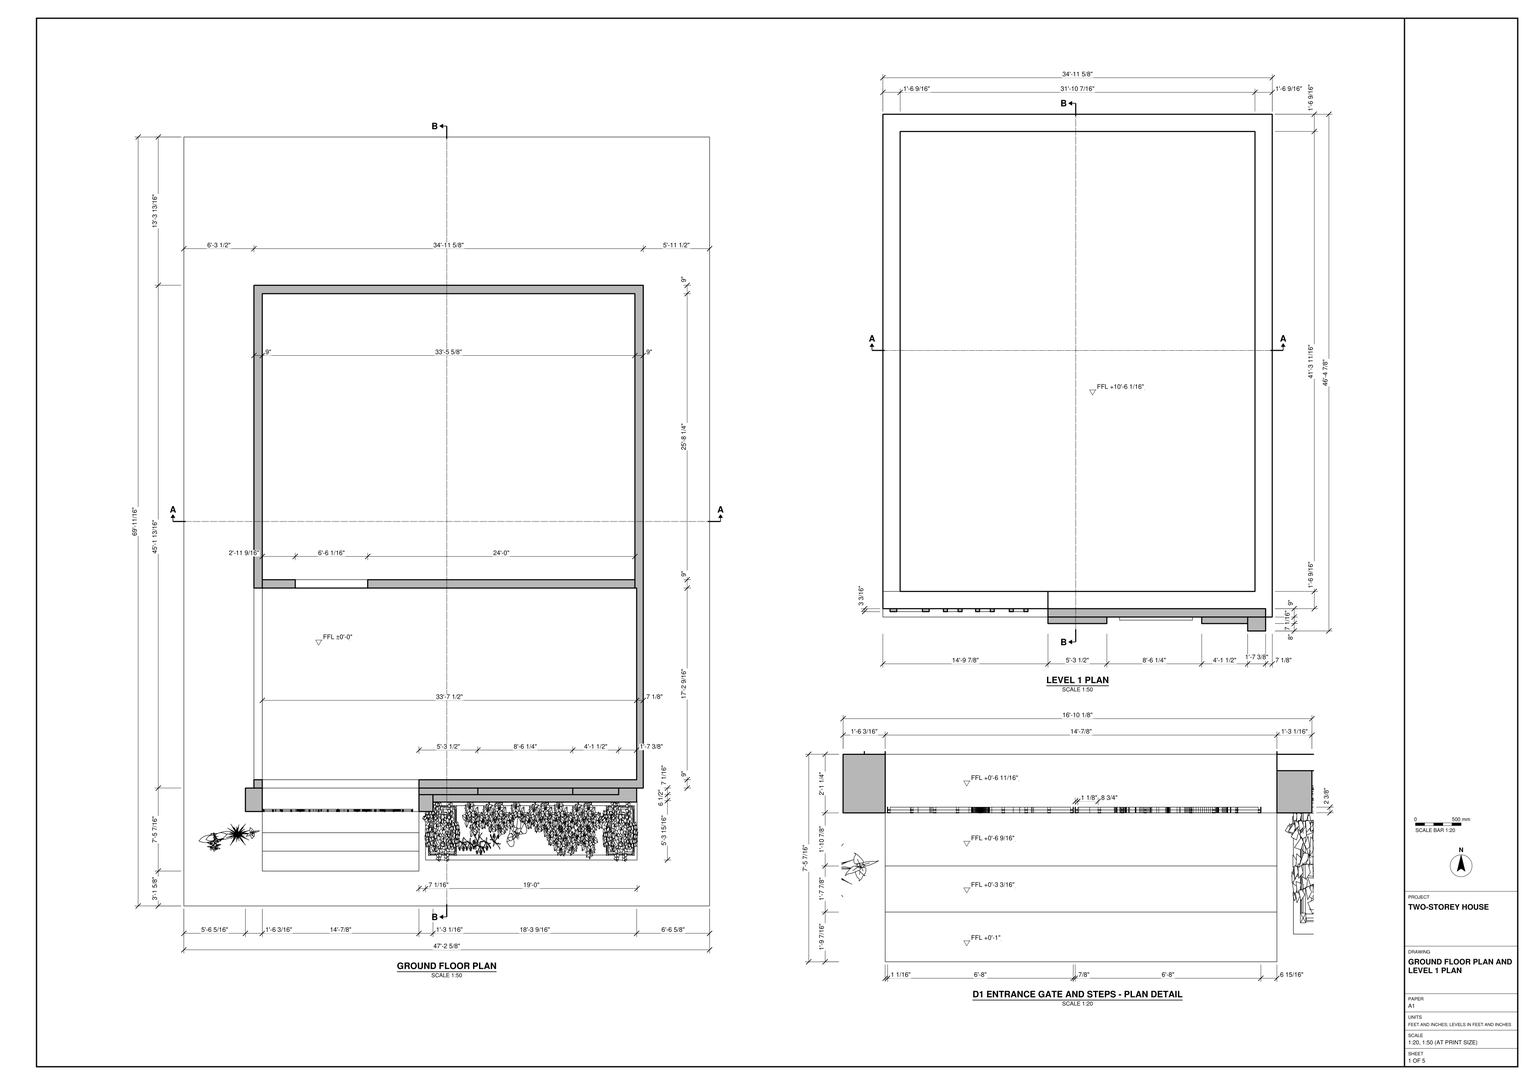
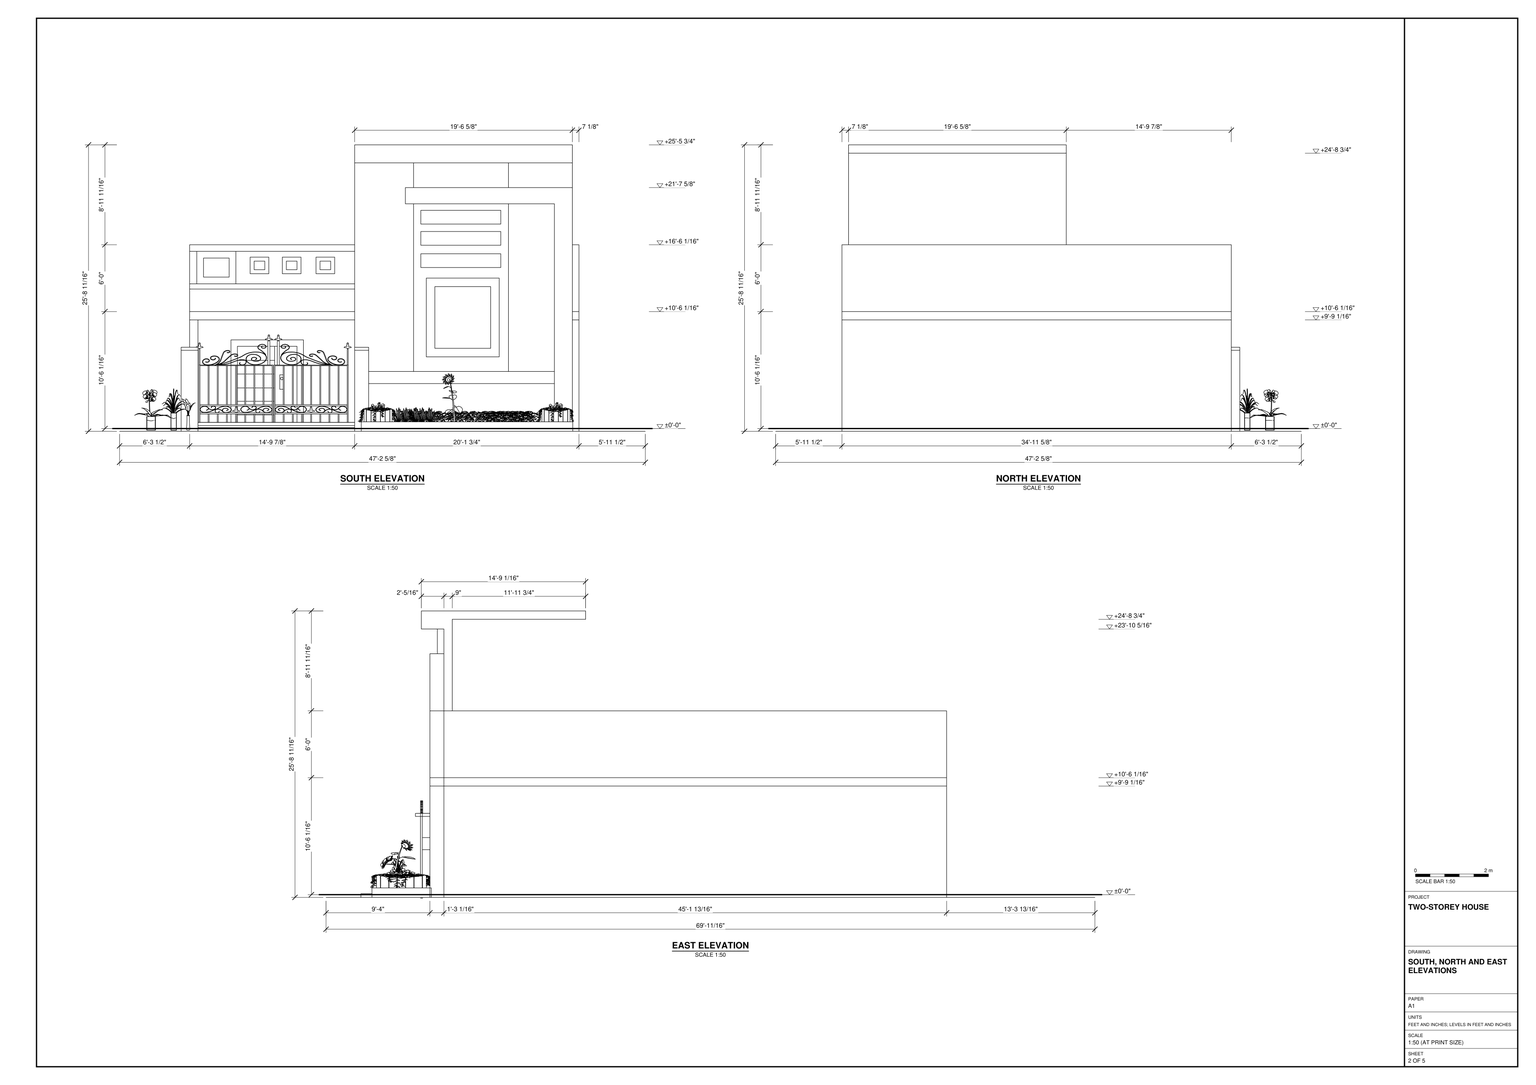
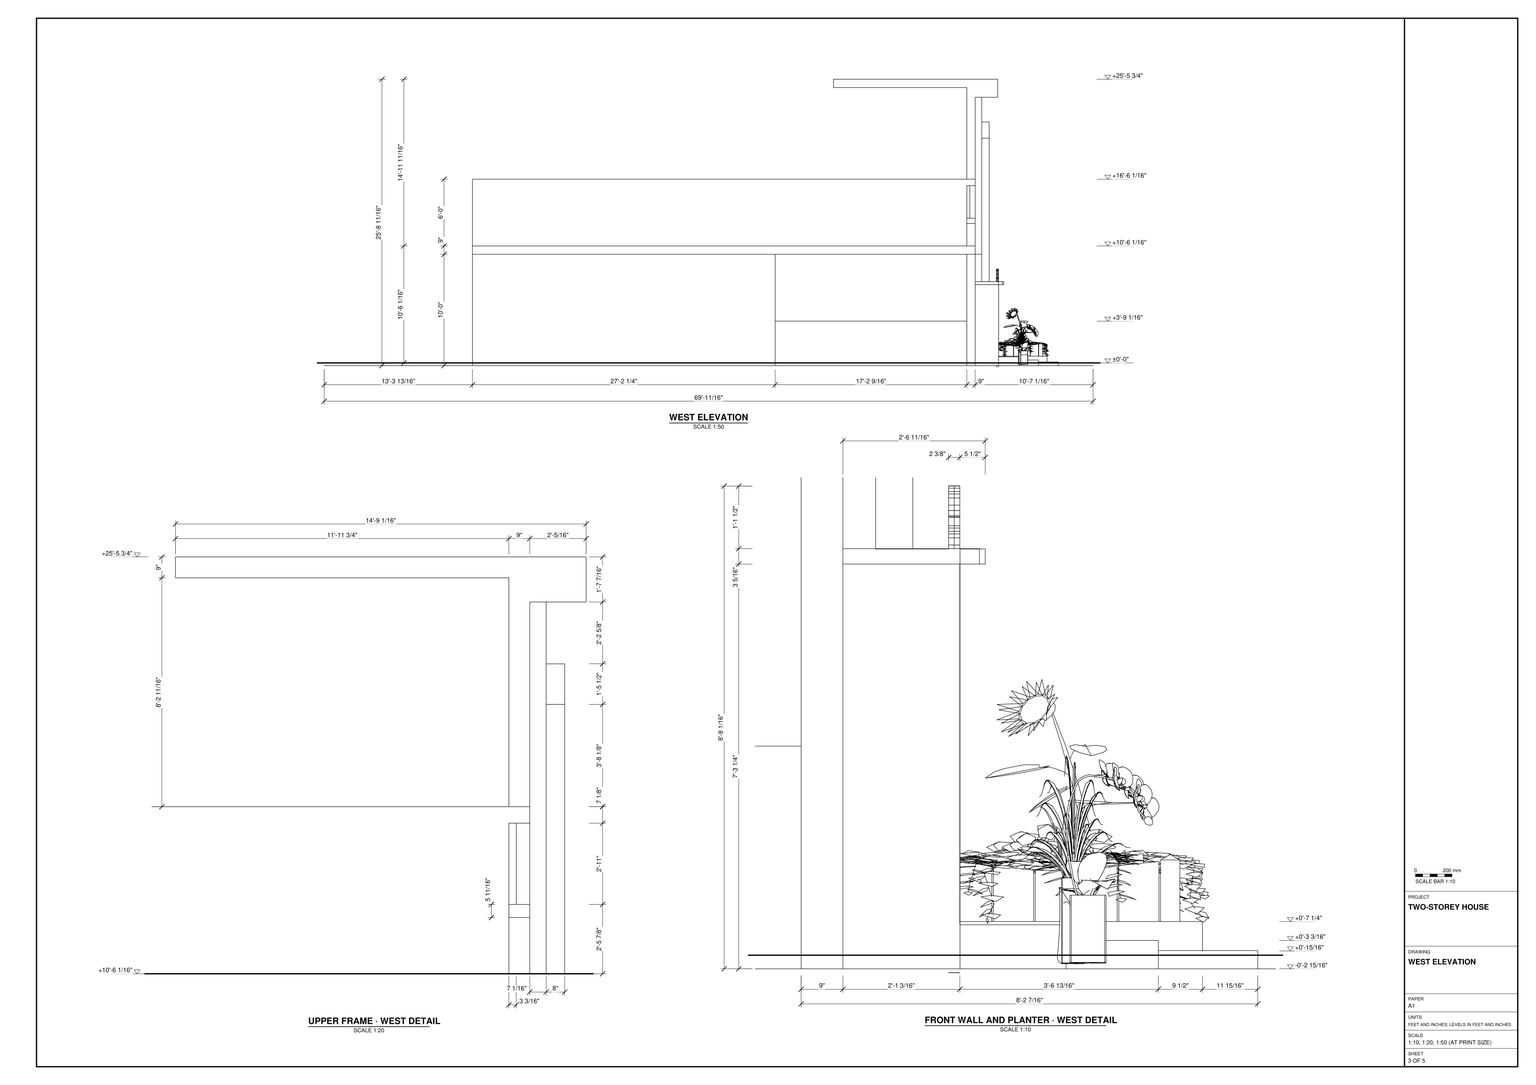
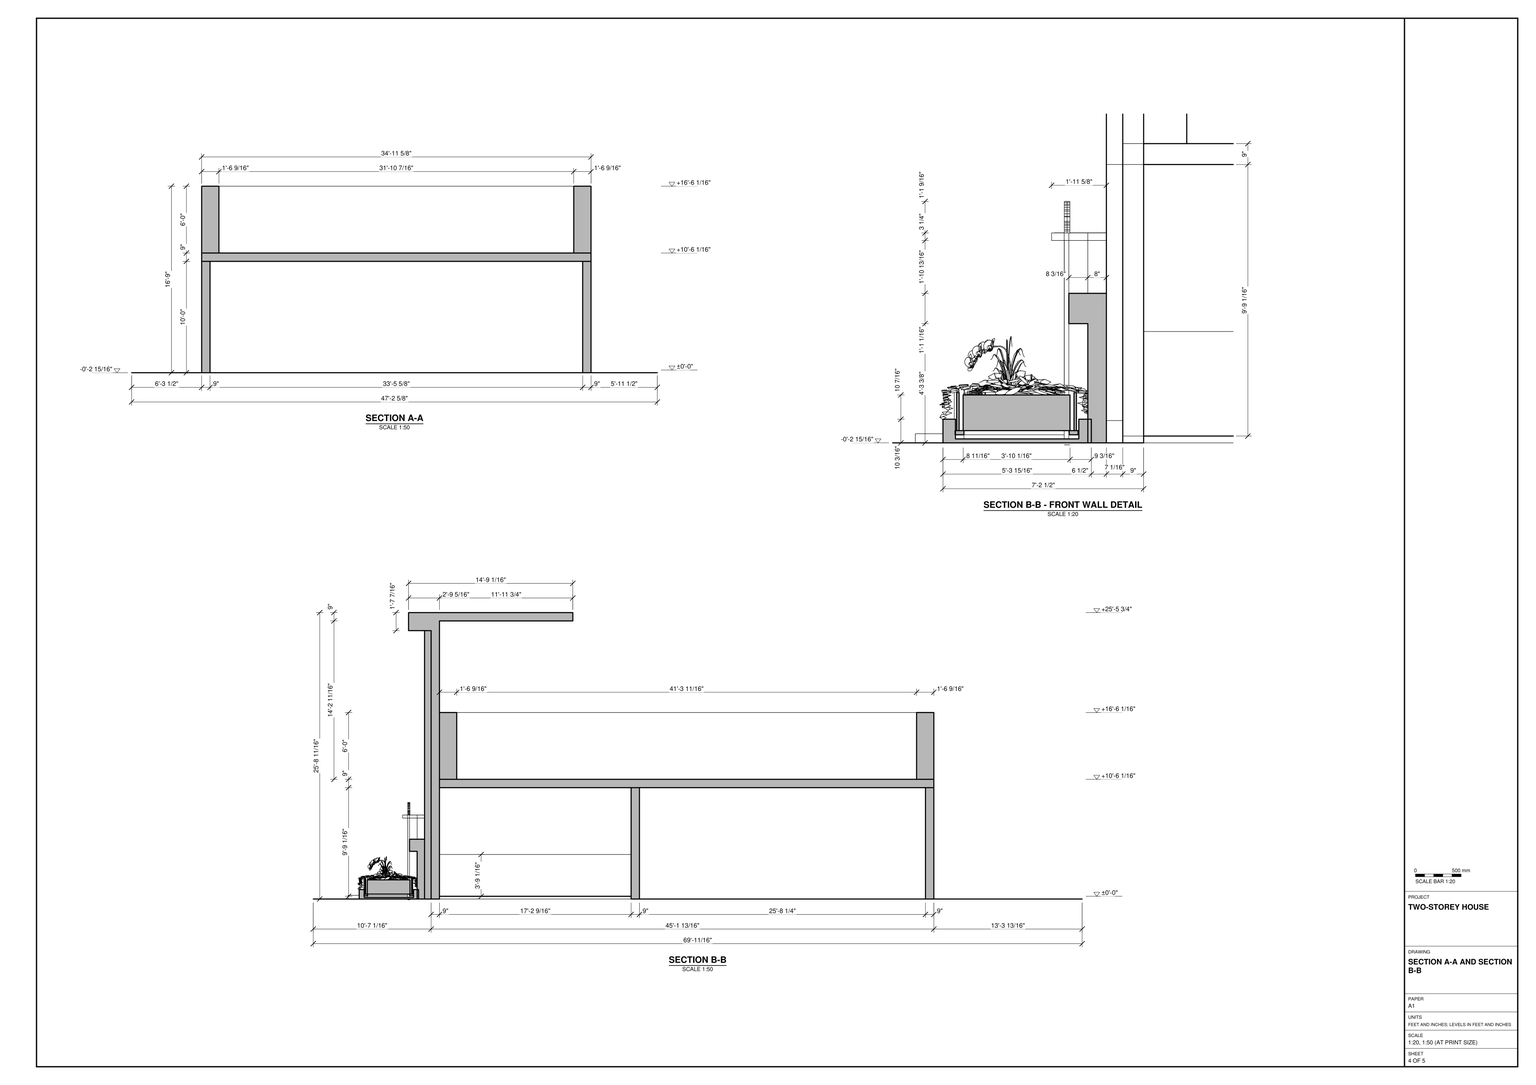
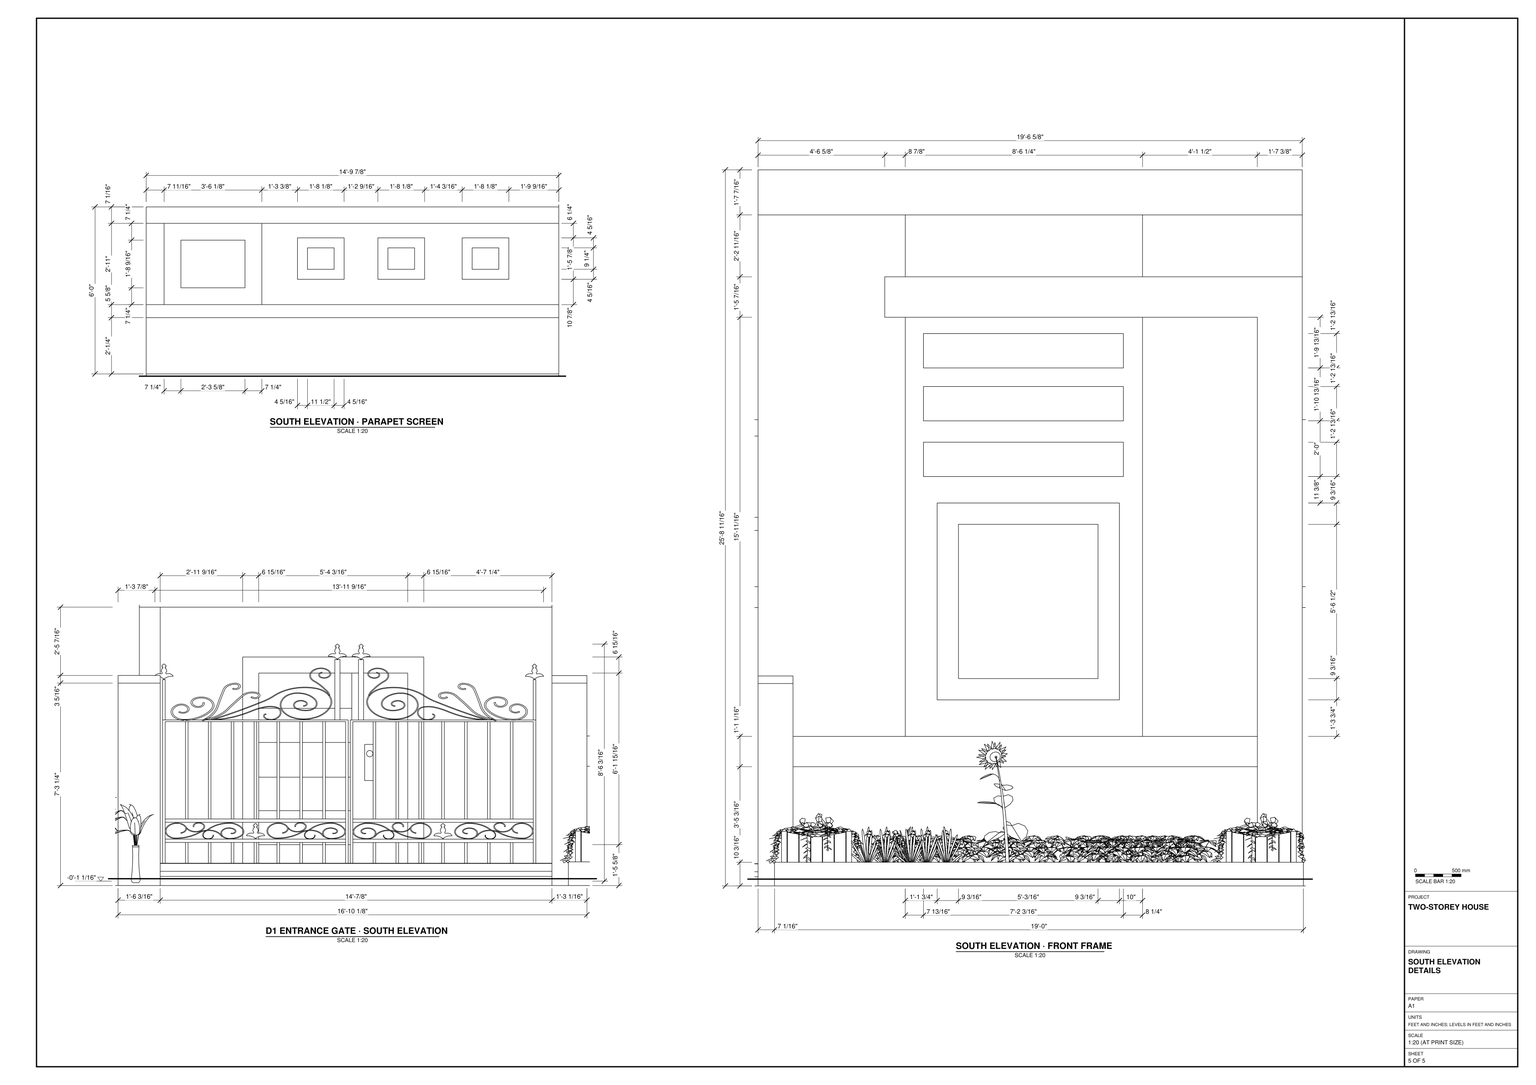
Build the house and its rectangular site in SketchUp from task_files/diagram_01.pdf. Work in feet and inches. The overall model is 47'-2 5/8" wide, 69'-11/16" deep and 25'-8 11/16" high. Set the ground floor at ±0'-0" and the upper floor at +10'-6 1/16".

Use the ground-floor plan to locate the house within the site. Model the rear enclosure, the cross wall with its offset doorway, and the entrance area in front of it. Follow the wall thicknesses as drawn, including the 9" walls around the rear enclosure. Form the upper slab and its raised perimeter, keeping the long side and rear elevations plain as shown.

Use the south elevation to set out the two different sides of the frontage. On the left, build the broad entrance steps, gateposts and paired gate leaves beneath the low band of framed panels. On the right, model the taller frame with its projecting flat roof, layered uprights, large framed panel and horizontal panels above. Use the west details to set the roof projection and the offsets between the front wall, planter and steps. Decor and loose items, including the planting, may be any suitable library components.

Keep walls, slabs, roof, gate and each furniture or joinery piece in separate groups or components, and use components for repeated parts. Save one SketchUp model as output_files/two_storey_house_with_a_stepped_entrance_and_front_gate.skp.

# SketchUp Ruby script. Lengths in inches.
U = 1.inch
M = Sketchup.active_model
def pt(a) = Geom::Point3d.new(a.map { |v| v * U })
def face(e, loops, mat)
  f = e.add_face(loops[0].map { |a| pt(a) })
  loops[1..].each { |l| e.add_face(l.map { |a| pt(a) }).erase! }
  f.material = f.back_material = mat if mat
  f
end
# faces: each face lists its corners as indices into pts; further lists are holes
def faces(e, pts, list, mat = nil) = list.each { |f| face(e, (f[0].is_a?(Array) ? f : [f]).map { |l| l.map { |i| pts[i] } }, mat) }
# xy, xz, yz: faces in a plane at the given z, y or x. An outline is a flat list of corners, or four numbers for a rectangle; further outlines are holes
def ring(l) = l.size == 4 ? [[l[0], l[1]], [l[2], l[1]], [l[2], l[3]], [l[0], l[3]]] : l.each_slice(2).to_a
def flat(e, list, mat, &to3) = list.each { |f| face(e, (f[0].is_a?(Array) ? f : [f]).map { |l| ring(l).map { |u, v| to3.(u, v) } }, mat) }
def xy(e, z, list, mat = nil) = flat(e, list, mat) { |x, y| [x, y, z] }
def xz(e, y, list, mat = nil) = flat(e, list, mat) { |x, z| [x, y, z] }
def yz(e, x, list, mat = nil) = flat(e, list, mat) { |y, z| [x, y, z] }
def lines(e, pts, list) = list.each { |a, b| e.add_line(pt(pts[a]), pt(pts[b])) }
# prism: a flat outline (further loops are holes) pulled along v
def prism(e, loops, v, mat = nil)
  f = face(e, loops, mat); d = Geom::Vector3d.new(v.map { |x| x * U })
  f.pushpull(f.normal.samedirection?(d) ? d.length : -d.length)
end
def box(e, o, s, mat = nil) = prism(e, [[o, [o[0] + s[0], o[1], o[2]], [o[0] + s[0], o[1] + s[1], o[2]], [o[0], o[1] + s[1], o[2]]]], [0, 0, s[2]], mat)
def at(x, y, z, deg = 0) = Geom::Transformation.translation(pt([x, y, z])) * Geom::Transformation.rotation(ORIGIN, Z_AXIS, deg.degrees)
def axes(o, x, y, z) = Geom::Transformation.new([*x, 0, *y, 0, *z, 0, *pt(o).to_a, 1])
def part(name) = M.definitions.add(name)
# library, detail: a bought-in or finely detailed component or shape, given as its bounding box
def library(name, o, s) = part(name).tap { |d| box(d.entities, o, s) }
def detail(e, o, s) = box(e.add_group.entities, o, s)
def put(e, d, t, mat = nil) = e.add_instance(d, t).tap { |i| i.material = mat if mat }
def group(e, t, mat = nil) = e.add_group.tap { |g| g.transformation = t; g.material = mat if mat }.entities
root = M.entities
M.materials.add("[Blinds Wood Natural]").color = [167, 145, 74]
M.materials.add("[Color C01]").color = [255, 229, 204]
M.materials.add("[Color C03]").color = [255, 178, 101]
M.materials.add("[Color C04]").color = [255, 153, 50]
M.materials.add("[Color D03]").color = [255, 216, 101]
M.materials.add("[Color D04]").color = [255, 204, 50]
M.materials.add("[Formica Graystone]").color = [149, 146, 135]
M.materials.add("[Formica Laminate Dark]").color = [50, 53, 60]
M.materials.add("[Formica Speckled Grey]").color = [94, 105, 111]
M.materials.add("[Translucent Glass Sky Reflection]").color = [126, 138, 183]
M.materials["[Translucent Glass Sky Reflection]"].alpha = 0.52
M.materials.add("[Wood Bamboo]").color = [177, 105, 43]
M.materials.add("[Wood Board Cork]").color = [215, 201, 115]
M.materials.add("[Wood Veneer 01]").color = [120, 70, 37]
M.materials.add("bottom").color = [37, 104, 50]
c1 = library("gate",[-17.08,19.83,-10.33],[162.44,1,145.04])
c2 = library("Planter_Wood_Square",[-12.51,-6.53,0],[58.51,52.32,45.58])
c3 = library("Plant_Sunflower",[-13.8,-15.43,0],[27.09,16.85,64.87])
c4 = part("Lg Broken Leaf")
p = [[0.72,6.4,1.375],[1.32,6.4,1.375],[1.31,6.44,1.32],[1.02,7.29,0],[0.73,6.44,1.32],[0.5,5.3,2.66],
  [1.54,5.3,2.66],[1.53,5.35,2.61],[1.4375,5.9,1.96],[0.6,5.9,1.96],[0.51,5.35,2.61],[0.44,4.6875,3.23],
  [0.41,4.02,3.84],[1.63,4.02,3.84],[1.6,4.6875,3.23],[0.43,2.57,4.9],[1.61,2.57,4.9],[1.63,3.22,4.43],
  [0.41,3.22,4.43],[0.65,0.97,5.83],[1.39,0.97,5.83],[1.47,1.4,5.58],[1.54,1.9,5.29],[1.6,2.41,5],
  [0.44,2.41,5],[0.5,1.9,5.29],[0.57,1.4,5.58],[1.02,0.33,6.11]]
faces(c4.entities,p,[[0,1,2,3,4],[5,6,7,8,1,0,9,10],[6,5,11,12,13,14],[15,16,17,13,12,18],[19,20,21,22,23,16,15,24,25,26],[19,27,20]],"bottom")
c5 = part("stalk")
xy(c5.entities,13.2,[[0.11,0.17,0.11,0.29,0,0.23]])
p = [[0.8,0,0],[0.3,0,7.2],[0.05,0.15,7.2],[0.64,0.09,0],[0.8,0.18,0],[0.3,0.29,7.2],
  [0.11,0.17,13.2],[0,0.23,13.2],[0.11,0.29,13.2]]
faces(c5.entities,p,[[0,1,2,3],[0,4,5,1],[3,2,5,4],[1,6,7,2],[1,5,8,6],[2,7,8,5]])
c6 = part("petal\#1")
p = [[0.62,0.42,-0.27],[0.71,0.28,-0.07],[0.72,0.84,-0.07],[0.62,0.7,-0.27],[1,0,0.21],[1,1.12,0.2],
  [1.53,1.12,0.4375],[1.53,0,0.4375],[1.53,0.56,0.4375],[1.99,0.28,0.3],[2.23,0.42,0.23],[2.23,0.7,0.22],
  [1.99,0.84,0.3],[1.76,0.79,0.37],[1.76,0.33,0.37]]
faces(c6.entities,p,[[0,1,2,3],[1,4,5,2],[6,5,4,7,8],[9,10,11,12,13,8,14],[14,8,7,9],[6,8,13,12]])
c7 = part("petal\#2")
p = [[1.12,0.18,-0.52],[1.09,-0.07,-0.2],[1.09,0.58,-0.2],[1.12,0.37,-0.52],[1.25,-0.26,0.16],[1.25,0.78,0.16],
  [1.64,0.81,0.44],[1.64,-0.23,0.44],[1.64,0.36,0.44],[1.875,0.2,0.36],[2.24,0,0.23],[2.34,0.26,0.2],
  [2.34,0.45,0.2],[2.08,0.61,0.29],[1.875,0.51,0.36]]
faces(c7.entities,p,[[0,1,2,3],[1,4,5,2],[6,5,4,7,8],[9,8,7,10],[10,11,12,13,14,8,9],[6,8,14,13]])
c8 = part("flower\#1")
put(c8.entities,c6,axes([2.11,0.17,0.22],[-0.04332,0.67288,0.31447],[-0.79297,-0.00158,-0.10584],[-0.09505,-0.34133,0.71726]))
put(c8.entities,c6,axes([1.96,3.15,0.77],[-0.34058,-0.53026,-0.04745],[0.67203,-0.43351,0.02099],[-0.07223,-0.05636,1.14835]))
put(c8.entities,c7,axes([1.875,2.15,2.86],[-0.19209,-0.10227,-0.76975],[0.18918,-0.78348,0.05688],[0.7612,0.16839,-0.21233]))
put(c8.entities,c7,axes([-0.27,1.75,2.2],[0.7458,-0.1672,-0.4029],[0.09529,0.84119,-0.17269],[-0.42568,-0.10463,-0.74454]))
put(c8.entities,c7,axes([1.35,1,3.03],[0.21021,0.29303,-0.80271],[-0.84848,0.16975,-0.16023],[-0.10149,-0.81223,-0.32308]))
put(c8.entities,c6,axes([-0.01,1.74,0.14],[0.65005,-0.20903,0.29542],[0.19101,0.76714,0.12251],[-0.33903,-0.0312,0.72394]))
c9 = part("flower all")
put(c9.entities,c5,axes([1.5,1.42,0],[1,0,0],[0,1,0],[0,0,0.95]))
put(c9.entities,c8,axes([-0.1875,-0.26,11.36],[1.15,0,0],[0,1.15,0],[0,0,1.15]))
c10 = part("Plant_Iris")
put(c10.entities,c4,axes([2.34,6.11,0.91],[-0.7307,0.19579,0],[-0.22806,-0.85114,-0.14272],[-0.13461,-0.50236,3.2111]))
put(c10.entities,c4,axes([-1.55,-5.13,1.15],[0.73882,-0.13929,-0.08363],[0.1194,0.7313,-0.16322],[0.43446,0.57278,2.88421]),"bottom")
put(c10.entities,c4,axes([2.25,3.63,0.45],[-0.67969,0.25481,0.21297],[-0.22484,-0.52301,-0.09181],[0.54964,-0.68886,2.5783]),"bottom")
put(c10.entities,c4,axes([0.97,5.42,1.15],[-0.75102,0.03511,-0.08363],[-0.01646,-0.7408,-0.16322],[-0.36512,-0.65382,3.00438]),"bottom")
put(c10.entities,c4,axes([-1.78,-3.31,-0.01],[0.47543,-0.10678,0.47549],[0.18828,0.47676,-0.08118],[-0.92661,0.54451,1.04877]),"bottom")
put(c10.entities,c9,axes([2.89,-2.41,-0.46],[-0.34687,1.29454,0.20029],[-1.30891,-0.35072,0],[0.05184,-0.19347,1.3402]))
put(c10.entities,c4,axes([-1.58,-3.78,0.45],[0.70854,-0.15773,0.21297],[0.14986,0.54921,-0.09181],[-0.64016,0.60566,2.5783]),"bottom")
put(c10.entities,c4,axes([1.58,3.45,1.03],[-0.55594,0.20323,-0.33638],[-0.13288,-0.49532,-0.07964],[-1.26871,0.00294,2.09858]),"bottom")
put(c10.entities,c4,axes([-1.84,-3.14,0.82],[0.51728,-0.26469,-0.35481],[0.18828,0.47676,-0.08118],[0.9646,-0.12552,1.4999]),"bottom")
put(c10.entities,c4,axes([-1.95,-3.09,0.74],[0.55657,-0.28236,-0.27208],[0.20053,0.47201,-0.07964],[1.04737,-0.07102,2.21622]),"bottom")
put(c10.entities,c9,axes([2.04,-1.8125,0.13],[-0.26709,0.99679,0.15423],[-0.97505,-0.21431,-0.30344],[-0.2582,-0.22179,0.98634]))
c11 = part("leaf\#2")
p = [[2.22,5.43,0.5],[2.22,4.99,0.65],[2.22,3.75,0.8],[2.22,1.875,0.75],[2.22,0,0.5]]
lines(c11.entities,p,[[0,1],[1,2],[2,3],[3,4]])
g1 = group(c11.entities,at(-0.85,1.38,-0.53))
p = [[1.95,0.49,1.28],[3.0625,-1.38,1.03],[4.17,0.49,1.28],[4.89,3.61,1.18],[3.0625,4.05,1.03],[1.23,3.61,1.18],
  [5.28,2.37,1.33],[0.85,2.37,1.33],[4.09,0.37,1.26],[3.0625,5.5,0.53]]
faces(g1,p,[[0,1,2],[3,4,5],[6,7,5,3],[6,2,0,7]])
lines(g1,p,[[2,8],[4,9]])
c12 = part("stem")
p = [[0.07,0.07,0],[0.18,-0.6,6.17],[0.15,-0.52,6.17],[0,0.23,0],[0.22,0,0],[0.26,-0.63,6.17],
  [0.38,0.07,0],[0.34,-0.6,6.17],[0.45,0.23,0],[0.375,-0.52,6.17],[0.18,-0.44,6.17],[0.07,0.38,0],
  [0.38,0.38,0],[0.34,-0.44,6.17],[0.22,0.45,0],[0.26,-0.41,6.17],[0.3,0.36,14.04],[0.3,0.37,14.04],
  [0.31,0.36,14.04],[0.32,0.37,14.04],[0.3125,0.36,14.04],[0.3,0.375,14.04],[0.3125,0.375,14.04],[0.31,0.375,14.04]]
faces(c12.entities,p,[[0,1,2,3],[0,4,5,1],[6,7,5,4],[6,8,9,7],[3,2,10,11],[8,12,13,9],[14,11,10,15],[14,15,13,12],
  [1,16,17,2],[1,5,18,16],[7,9,19,20],[7,20,18,5],[2,17,21,10],[9,13,22,19],[15,10,21,23],[15,23,22,13]])
c13 = part("Plant_Copperleaf")
put(c13.entities,c11,axes([-5.58,4.88,9.66],[0.029,-0.6438,-0.08473],[0.46185,-0.03917,0.4557],[-0.45646,-0.08053,0.4557]))
put(c13.entities,c11,axes([-5.08,1.59,6.46],[0.32516,-0.5592,0.06373],[0.34931,0.25823,0.48353],[-0.4413,-0.20764,0.4297]))
put(c13.entities,c11,axes([1.03,7.88,12.84],[-0.74201,0.41464,0],[-0.35359,-0.63275,0.44396],[0.21657,0.38756,0.72484]))
put(c13.entities,c11,axes([8.15,-2.85,6.5],[0.20357,0.97906,0],[-0.82181,0.17088,0.54354],[0.53216,-0.11065,0.83938]))
put(c13.entities,c11,axes([-2.45,-8.68,11.21],[0.44862,0.69737,0.18686],[-0.68348,0.33936,0.37442],[0.23259,-0.34787,0.73986]))
put(c13.entities,c11,axes([5.75,-5.02,11.05],[0.73612,0.3986,0.14745],[-0.425,0.6904,0.25539],[0,-0.2949,0.79721]))
put(c13.entities,c11,axes([-9.53,-8.18,10.32],[0.69881,-0.44455,0.19116],[0.26519,0.63267,0.5019],[-0.40477,-0.35298,0.65883]))
put(c13.entities,c11,axes([-3.54,0.82,12.95],[0.59529,0.24687,-0.08473],[-0.12073,0.44751,0.4557],[0.23141,-0.40161,0.4557]))
put(c13.entities,c11,axes([-7.83,6.75,12.84],[-0.07243,-0.84691,0],[0.72233,-0.06177,0.44377],[-0.44215,0.03781,0.72496]))
put(c13.entities,c11,axes([5.33,5.4,7.18],[-0.82339,0.16353,0.1334],[-0.08131,-0.74163,0.40728],[0.19475,0.38176,0.73405]))
put(c13.entities,c11,axes([1.24,4.74,6.1875],[-0.56984,-0.3127,0],[0.2731,-0.49769,0.31658],[-0.1523,0.27754,0.56769]))
put(c13.entities,c11,axes([-7.98,-0.98,12.17],[-0.32199,-0.5173,-0.22633],[0.3682,-0.38989,0.3673],[-0.42807,0.05375,0.48617]))
put(c13.entities,c11,axes([-6.29,1.25,4.06],[0.17169,-0.81932,0.14745],[0.70535,0.22313,0.41856],[-0.44215,0.03781,0.72496]))
put(c13.entities,c11,axes([1.45,5.96,12.73],[-0.5734,-0.62614,-0.04073],[0.6224,-0.57457,0.07055],[-0.07951,0.01777,0.84609]))
put(c13.entities,c11,axes([2.15,3.51,2.68],[-0.74201,0.41464,0],[-0.26708,-0.47794,0.65018],[0.31717,0.56758,0.54751]))
put(c13.entities,c11,axes([-1.77,-7.74,6.875],[0.58011,0.60352,0.14745],[-0.5818,0.45697,0.41856],[0.21792,-0.38658,0.72496]))
put(c13.entities,c11,axes([4.56,3.08,6.68],[-0.50822,0.85524,-0.10132],[-0.77037,-0.39886,0.49743],[0.38501,0.33086,0.86157]))
put(c13.entities,c11,axes([-1.36,-1.16,13.02],[-0.63498,0.48874,0.28361],[-0.49336,-0.68751,0.08018],[0.27549,-0.10472,0.79727]))
put(c13.entities,c12,axes([-0.77,0.55,5.03],[0.06901,0.68185,-0.0317],[-0.56289,0.07487,0.38502],[0.38611,-0.01272,0.56696]))
put(c13.entities,c11,axes([-1.01,-0.89,8.07],[-0.53939,0.35267,-0.08473],[-0.34351,-0.44796,0.32223],[0.11644,0.31217,0.55811]))
put(c13.entities,c11,axes([6.98,3.76,4.09],[-0.72792,0.66854,0.15229],[-0.49329,-0.66488,0.56089],[0.47623,0.33316,0.81376]))
put(c13.entities,c11,axes([-1.09,-1.24,11.25],[0.51443,-0.67666,0],[0.64058,0.487,0.27383],[-0.21799,-0.16573,0.80468]))
put(c13.entities,c11,axes([8.08,1.18,10.18],[-0.40665,0.49996,-0.08473],[-0.39437,-0.24354,0.4557],[0.31876,0.3365,0.4557]))
put(c13.entities,c11,axes([-9.63,-1.83,7.02],[0.07558,-0.84663,0],[0.72197,0.06445,0.44396],[-0.4422,-0.03947,0.72484]))
put(c13.entities,c11,axes([2.71,-1.18,1.48],[0.27025,0.73847,0.14708],[-0.41941,0.01785,0.68101],[0.62535,-0.30716,0.39318]))
put(c13.entities,c12,axes([-0.27,-0.29,-0.05],[1.17914,0.05766,0.21521],[0,1.15911,-0.31058],[-0.2228,0.30518,1.13896]))
put(c13.entities,c11,axes([1.52,0.375,4.23],[-0.45629,0.46292,0.00108],[-0.43266,-0.427,0.23018],[0.16464,0.16086,0.60788]))
put(c13.entities,c11,axes([-7.16,-2.94,2.12],[0.60544,-0.58565,-0.11382],[0.48786,0.39265,0.57473],[-0.34341,-0.4747,0.61582]))
put(c13.entities,c11,axes([-3.79,3.68,3.05],[-0.44676,-0.6045,-0.39686],[0.31657,-0.58291,0.53151],[-0.65015,0.13155,0.53151]))
put(c13.entities,c11,axes([-0.3,8.01,9.4],[-0.82874,0.11809,0.14745],[-0.03086,-0.73916,0.41856],[0.18637,0.40274,0.72496]))
put(c13.entities,c12,axes([-0.79,0.44,2.66],[0.65559,-0.72856,0],[0.60007,0.53997,0.55583],[-0.41317,-0.3718,0.80725]))
put(c13.entities,c11,axes([2.6875,-5.36,4.22],[0.87183,0.48981,0],[-0.39311,0.69971,0.59654],[0.29219,-0.52008,0.80258]))
put(c13.entities,c11,axes([0.09,-5.84,2.26],[0.61933,0.36626,0.45253],[-0.57159,0.50795,0.37117],[-0.11049,-0.57475,0.61641]))
put(c13.entities,c11,axes([-0.51,-1.82,9.55],[0.64288,0.55606,0],[-0.47418,0.54822,0.44396],[0.29044,-0.33578,0.72484]))
put(c13.entities,c11,axes([-3.38,7.24,4.89],[-0.76712,-0.64061,0.03388],[0.46704,-0.52151,0.71407],[-0.43977,0.5636,0.69925]))
c14 = part("Group\#6")
put(c14.entities,c13,at(38.08,13.93,0.15,57.3))
put(c14.entities,c13,at(8.91,14.4,0.15,95.1))
put(c14.entities,c13,at(27.59,12.47,0.15,84.3))
put(c14.entities,c13,at(47.4,9.34,0.15))
put(c14.entities,c13,at(17.4,9.34,0.15))
c15 = part("sledgegarden")
xy(c15.entities,0,[[-83.88,-7.53,144.12,28.47]])
xy(c15.entities,2,[[-80.85,-4.5,-50.62,25.4375],[110.87,-4.5,141.09,25.4375]])
xy(c15.entities,9.5,[[-50.62,-4.5,110.87,25.4375]])
xy(c15.entities,12,[[[-83.88,-7.53,144.12,28.47],[-80.85,-4.5,141.09,25.4375]]])
xz(c15.entities,-7.53,[[-83.88,0,144.12,12]])
xz(c15.entities,-4.5,[[-80.85,2,-80.85,12,141.09,12,141.09,2,110.87,2,110.87,9.5,-50.62,9.5,-50.62,2]])
xz(c15.entities,25.4375,[[-80.85,2,-50.62,2,-50.62,9.5,110.87,9.5,110.87,2,141.09,2,141.09,12,-80.85,12]])
xz(c15.entities,28.47,[[-83.88,0,144.12,12]])
yz(c15.entities,-83.88,[[-7.53,0,28.47,12]])
yz(c15.entities,-80.85,[[-4.5,2,25.4375,12]])
yz(c15.entities,-50.62,[[-4.5,2,25.4375,9.5]])
yz(c15.entities,110.87,[[-4.5,2,25.4375,9.5]])
yz(c15.entities,141.09,[[-4.5,2,25.4375,12]])
yz(c15.entities,144.12,[[-7.53,0,28.47,12]])
put(c15.entities,c2,axes([-80.85,-4.79,2],[0.78,0,0],[0,0.78,0],[0,0,0.78]))
put(c15.entities,c2,axes([110.87,-4.79,2],[0.78,0,0],[0,0.78,0],[0,0,0.78]))
put(c15.entities,c3,at(16.73,5.08,9.5,-153.1))
put(c15.entities,c10,at(-43.9375,2.89,9.5))
put(c15.entities,c10,at(-36.1875,2.89,9.5))
put(c15.entities,c10,at(-27.87,3.31,9.64,-105))
put(c15.entities,c10,at(-18.57,3.27,9.64))
put(c15.entities,c10,at(-9.69,3.48,9.64,171.1))
put(c15.entities,c10,at(-25.13,0.73,9.5))
put(c15.entities,c14,at(51.73,6.4,9.49))
put(c15.entities,c14,at(5.35,6.4,9.49))
put(c15.entities,c14,at(-44.32,6.4,9.49))
put(c15.entities,c14,at(101.8,16.28,9.49,180))
c16 = library("plantas+internas",[0,0,0],[44.91,27.47,36.11])
xy(root,0,[[[0,0,566.625,828.6875],[84.5,37.6,253.38,37.6,253.38,101.79,268.46,101.79,268.46,111.98,488,111.98,488,127.04,495.125,127.04,495.125,668.875,75.5,668.875,75.5,127.04,66.34,127.04,66.34,101.79,84.5,101.79]],[84.5,37.6,253.38,59.04],[84.5,59.04,253.38,78.91],[84.5,78.91,253.38,101.79],[66.34,101.79,84.5,127.04],
  [84.5,101.79,253.38,127.04],[253.38,101.79,268.46,119.98],[268.46,111.98,268.46,119.98,468.64,119.98,468.64,127.04,488,127.04,488,111.98],[253.38,119.98,316.86,127.04],[419.14,119.98,468.64,127.04],
  [253.38,127.04,253.38,136.04,488,136.04,488,342.6,486.125,342.6,486.125,659.875,84.5,659.875,84.5,342.6,75.5,342.6,75.5,668.875,495.125,668.875,495.125,127.04],[75.5,127.04,84.5,136.04],[84.5,127.04,253.38,136.04],[75.5,136.04,84.5,342.6],[84.5,342.6,120.0625,351.6],
  [198.125,342.6,486.125,351.6],[84.5,351.6,486.125,659.875]])
xy(root,2.9375,[[84.5,127.04,253.38,136.04],[120.0625,342.6,198.125,351.6]])
xy(root,2.9375,[[84.5,136.04,488,342.6]],"[Formica Graystone]")
xy(root,3.9375,[[84.5,37.6,253.38,59.04]],"[Formica Graystone]")
xy(root,6.125,[[84.5,59.04,253.38,78.91]],"[Formica Graystone]")
xy(root,9.5,[[84.5,78.91,253.38,101.79]],"[Formica Graystone]")
xy(root,9.625,[[84.5,101.79,253.38,127.04]],"[Formica Graystone]")
xy(root,48,[[75.5,136.04,84.5,342.6]],"[Color C03]")
xy(root,51.4,[[268.46,103.79,468.64,111.98]],"[Color C04]")
xy(root,64.46,[[268.46,103.79,468.64,119.98]],"[Color D03]")
xy(root,80.19,[[330.59,123.66,409.15,127.04]])
xy(root,87.25,[[253.38,96.35,268.46,101.79],[66.34,97.6,84.5,101.79],[66.34,101.79,84.5,127.04],[253.38,101.79,268.46,119.98]])
xy(root,89.39,[[339.79,123.66,399.96,127.04]])
xy(root,90.5,[[253.38,96.35,268.46,101.79],[253.38,101.79,268.46,119.98]],"[Color D03]")
xy(root,90.5625,[[66.34,97.6,84.5,101.79],[66.34,101.79,84.5,127.04]],"[Color D03]")
xy(root,98.5,[[120.0625,342.6,198.125,351.6]])
xy(root,120,[[488,127.04,488,342.6,486.125,342.6,486.125,659.875,84.5,659.875,84.5,342.6,75.5,342.6,75.5,668.875,495.125,668.875,495.125,127.04],[75.5,127.04,84.5,136.04],[84.5,342.6,486.125,351.6],[84.5,342.6,486.125,659.875]])
xy(root,120,[[84.5,127.04,84.5,136.04,75.5,136.04,75.5,342.6,488,342.6,488,136.04,253.38,136.04,253.38,127.04]],"[Color D04]")
xy(root,129,[[488,127.04,488,136.04,253.38,136.04,253.38,154.625,476.54,154.625,476.54,650.29,94.09,650.29,94.09,154.625,75.5,154.625,75.5,668.875,495.125,668.875,495.125,127.04],[75.5,136.04,253.38,154.625],[94.09,154.625,476.54,650.29]])
xy(root,129,[[75.5,127.04,253.38,136.04]],"[Color C03]")
xy(root,153.25,[[75.5,127.04,253.38,136.04]])
xy(root,155.87,[[339.79,123.66,399.96,127.04]])
xy(root,158.88,[[83.21,132.85,125.36,136.04]])
xy(root,158.88,[[75.5,127.04,253.38,127.04,253.38,136.04,125.36,136.04,125.36,132.85,83.21,132.85,83.21,136.04,75.5,136.04]],"[Color C03]")
xy(root,165.07,[[330.59,123.66,409.15,127.04]])
xy(root,166.13,[[90.46,132.85,118.11,136.04]])
xy(root,169.79,[[140.72,132.85,160.84,136.04],[175.4,132.85,195.53,136.04],[211.72,132.85,231.84,136.04]])
xy(root,174.1,[[145.03,132.85,156.53,136.04],[179.72,132.85,191.21,136.04],[216.03,132.85,227.53,136.04]])
xy(root,176.47,[[324.69,124.79,410.88,127.04]])
xy(root,183.35,[[145.03,132.85,156.53,136.04],[179.72,132.85,191.21,136.04],[216.03,132.85,227.53,136.04]])
xy(root,186.66,[[90.46,132.85,118.11,136.04]])
xy(root,187.66,[[140.72,132.85,160.84,136.04],[175.4,132.85,195.53,136.04],[211.72,132.85,231.84,136.04]])
xy(root,191.28,[[324.69,124.79,410.88,127.04]])
xy(root,193.91,[[75.5,127.04,75.5,136.04,83.21,136.04,83.21,132.85,125.36,132.85,125.36,136.04,253.38,136.04,253.38,127.04],[83.21,132.85,125.36,136.04]])
xy(root,200.47,[[324.69,124.79,410.88,127.04]])
xy(root,201,[[[75.5,127.04,253.38,127.04,253.38,136.04,488,136.04,488,127.04,495.125,127.04,495.125,668.875,75.5,668.875],[94.09,154.625,476.54,650.29]]],"[Color C03]")
xy(root,215.28,[[324.69,124.79,410.88,127.04]])
xy(root,223.28,[[324.69,124.79,410.88,127.04]])
xy(root,238.1,[[324.69,124.79,410.88,127.04]])
xy(root,245.125,[[308.01,111.98,316.86,119.98],[316.86,111.98,419.14,127.04],[419.14,111.98,468.64,119.98],[308.01,119.98,316.86,127.04],[419.14,119.98,468.64,127.04]])
xy(root,262.58,[[308.01,111.98,316.86,119.98],[316.86,111.98,419.14,127.04],[419.14,111.98,488,119.98],[308.01,119.98,316.86,127.04],[419.14,119.98,488,127.04]])
xy(root,289.25,[[253.38,102.73,253.38,119.98,316.86,119.98,316.86,127.04,419.14,127.04,419.14,119.98,488,119.98,488,102.73],[253.38,119.98,316.86,127.04],[419.14,119.98,488,127.04]])
xy(root,299.6875,[[253.38,136.04,488,279.79]])
xy(root,308.6875,[[253.38,102.73,488,279.79]],"[Color D03]")
xz(root,37.6,[[84.5,0,253.38,3.9375]],"[Formica Graystone]")
xz(root,59.04,[[84.5,0,253.38,3.9375]])
xz(root,59.04,[[84.5,3.9375,253.38,6.125]],"[Formica Graystone]")
xz(root,78.91,[[84.5,0,253.38,6.125]])
xz(root,78.91,[[84.5,6.125,253.38,9.5]],"[Formica Graystone]")
xz(root,96.35,[[253.38,87.25,268.46,90.5]],"[Color D03]")
xz(root,97.6,[[66.34,87.25,84.5,90.5625]],"[Color D03]")
xz(root,101.79,[[84.5,0,253.38,9.5],[84.5,9.5,253.38,9.625],[66.34,87.25,84.5,90.5625],[253.38,87.25,268.46,90.5]])
xz(root,101.79,[[66.34,0,84.5,87.25],[253.38,0,268.46,87.25]],"[Color D03]")
xz(root,102.73,[[253.38,289.25,488,308.6875]],"[Color D03]")
xz(root,103.79,[[268.46,51.4,468.64,64.46]],"[Color C04]")
xz(root,111.98,[[268.46,0,468.64,51.4]],"[Blinds Wood Natural]")
xz(root,111.98,[[468.64,0,488,0,488,262.58,308.01,262.58,308.01,245.125,468.64,245.125]],"[Color C04]")
xz(root,119.98,[[253.38,0,268.46,87.25],[316.86,0,419.14,64.46],[253.38,87.25,268.46,90.5]])
xz(root,119.98,[[419.14,0,468.64,64.46],[419.14,64.46,468.64,245.125],[419.14,262.58,488,289.25]],"[Blinds Wood Natural]")
xz(root,119.98,[[268.46,0,316.86,64.46],[268.46,64.46,316.86,64.46,316.86,245.125,308.01,245.125,308.01,262.58,316.86,262.58,316.86,289.25,253.38,289.25,253.38,90.5,268.46,90.5]],"[Formica Speckled Grey]")
xz(root,123.66,[[[330.59,80.19,409.15,165.07],[339.79,89.39,399.96,155.87]]])
xz(root,124.79,[[324.69,176.47,410.88,191.28],[324.69,200.47,410.88,215.28],[324.69,223.28,410.88,238.1]],"[Formica Laminate Dark]")
xz(root,127.04,[[66.34,0,75.5,87.25],[75.5,0,84.5,87.25],[84.5,0,253.38,2.9375],[253.38,0,253.38,289.25,316.86,289.25,316.86,262.58,308.01,262.58,308.01,245.125,316.86,245.125,316.86,0],[468.64,0,468.64,245.125,308.01,245.125,308.01,262.58,488,262.58,488,0],
  [419.14,0,468.64,245.125],[84.5,2.9375,253.38,9.625],[[330.59,80.19,409.15,165.07],[339.79,89.39,399.96,155.87]],[66.34,87.25,75.5,90.5625],[75.5,87.25,84.5,90.5625],
  [324.69,176.47,410.88,191.28],[324.69,200.47,410.88,215.28],[324.69,223.28,410.88,238.1],[419.14,262.58,488,289.25]])
xz(root,127.04,[[75.5,90.5625,84.5,120],[75.5,120,253.38,129],[75.5,153.25,253.38,158.88],[75.5,193.91,253.38,201]],"[Color C03]")
xz(root,127.04,[[[316.86,0,419.14,245.125],[330.59,80.19,409.15,165.07],[324.69,223.28,410.88,238.1],[324.69,200.47,410.88,215.28],[324.69,176.47,410.88,191.28]],[316.86,262.58,419.14,289.25]],"[Color C04]")
xz(root,127.04,[[488,0,495.125,120],[488,120,495.125,129],[488,129,495.125,201]],"[Color D03]")
xz(root,127.04,[[339.79,89.39,399.96,155.87]],"[Translucent Glass Sky Reflection]")
xz(root,132.85,[[[140.72,169.79,160.84,187.66],[145.03,174.1,156.53,183.35]],[[175.4,169.79,195.53,187.66],[179.72,174.1,191.21,183.35]],[[211.72,169.79,231.84,187.66],[216.03,174.1,227.53,183.35]]],"[Color C01]")
xz(root,132.85,[[[83.21,158.88,125.36,193.91],[90.46,166.13,118.11,186.66]]],"[Color C04]")
xz(root,136.04,[[75.5,0,84.5,48],[84.5,0,253.38,2.9375],[253.38,0,488,2.9375],[75.5,48,84.5,120],[253.38,120,488,129],
  [253.38,129,488,201],[75.5,153.25,253.38,158.88],[[83.21,158.88,125.36,193.91],[90.46,166.13,118.11,186.66]],[[140.72,169.79,160.84,187.66],[145.03,174.1,156.53,183.35]],[[175.4,169.79,195.53,187.66],[179.72,174.1,191.21,183.35]],
  [[211.72,169.79,231.84,187.66],[216.03,174.1,227.53,183.35]],[145.03,174.1,156.53,183.35],[179.72,174.1,191.21,183.35],[216.03,174.1,227.53,183.35],[253.38,201,488,299.6875]])
xz(root,136.04,[[75.5,129,253.38,153.25]],"[Blinds Wood Natural]")
xz(root,136.04,[[253.38,2.9375,488,120]],"[Color C03]")
xz(root,136.04,[[75.5,158.88,83.21,193.91],[[125.36,158.88,253.38,193.91],[140.72,169.79,160.84,187.66],[175.4,169.79,195.53,187.66],[211.72,169.79,231.84,187.66]]],"[Color C04]")
xz(root,136.04,[[90.46,166.13,118.11,186.66]],"[Color D03]")
xz(root,154.625,[[94.09,129,253.38,201],[253.38,129,476.54,201]])
xz(root,279.79,[[253.38,299.6875,488,308.6875]],"[Color D03]")
xz(root,342.6,[[75.5,0,84.5,48],[84.5,0,120.0625,2.9375],[198.125,0,486.125,2.9375],[486.125,0,488,2.9375],[486.125,2.9375,488,120]])
xz(root,342.6,[[84.5,2.9375,120.0625,2.9375,120.0625,98.5,198.125,98.5,198.125,2.9375,486.125,2.9375,486.125,120,84.5,120],[75.5,48,84.5,120]],"[Color C03]")
xz(root,342.6,[[126.99,2.9375,167.1,17.61],[[167.1,2.9375,191.2,91.58],[172.65,45.27,177.4,60.83]],[126.99,17.61,167.1,32.28],[126.99,32.28,167.1,46.7],[126.99,46.7,167.1,61.68],
  [126.99,61.68,167.1,76.38],[126.99,76.38,167.1,91.58]],"[Wood Bamboo]")
xz(root,342.6,[[[172.65,45.27,177.4,60.83],[174.82,55.48,174.46,55.53,174.13,55.67,173.84,55.88,173.625,56.17,173.49,56.5,173.44,56.86,173.49,57.21,173.625,57.54,173.84,57.83,174.13,58.05,174.46,58.18,174.82,58.23,175.17,58.18,175.5,58.05,175.79,57.83,176.01,57.54,176.14,57.21,176.19,56.86,176.14,56.5,176.01,56.17,175.79,55.88,175.5,55.67,175.17,55.53]],[174.82,55.48,175.17,55.53,175.5,55.67,175.79,55.88,176.01,56.17,176.14,56.5,176.19,56.86,176.14,57.21,176.01,57.54,175.79,57.83,175.5,58.05,175.17,58.18,174.82,58.23,174.46,58.18,174.13,58.05,173.84,57.83,173.625,57.54,173.49,57.21,173.44,56.86,173.49,56.5,173.625,56.17,173.84,55.88,174.13,55.67,174.46,55.53]],"[Wood Board Cork]")
xz(root,342.6,[[120.0625,2.9375,126.99,2.9375,126.99,91.58,191.2,91.58,191.2,2.9375,198.125,2.9375,198.125,98.5,120.0625,98.5]],"[Wood Veneer 01]")
xz(root,351.6,[[84.5,0,84.5,120,486.125,120,486.125,0,198.125,0,198.125,98.5,120.0625,98.5,120.0625,0],[120.0625,0,198.125,2.9375]])
xz(root,650.29,[[94.09,129,476.54,201]])
xz(root,659.875,[[84.5,0,486.125,120]])
xz(root,668.875,[[75.5,0,495.125,120],[75.5,120,495.125,129],[75.5,129,495.125,201]],"[Color D03]")
yz(root,66.34,[[101.79,0,127.04,87.25],[97.6,87.25,101.79,90.5625],[101.79,87.25,127.04,90.5625]],"[Color D03]")
yz(root,75.5,[[127.04,153.25,136.04,158.88]])
yz(root,75.5,[[127.04,0,136.04,120],[136.04,0,342.6,48],[342.6,0,668.875,120],[127.04,120,668.875,129],[136.04,129,136.04,193.91,127.04,193.91,127.04,201,668.875,201,668.875,129]],"[Color D03]")
yz(root,83.21,[[132.85,158.88,136.04,193.91]])
yz(root,84.5,[[101.79,0,127.04,9.625],[127.04,0,136.04,2.9375],[136.04,0,342.6,2.9375],[342.6,0,351.6,120],[351.6,0,659.875,120]])
yz(root,84.5,[[127.04,2.9375,136.04,120],[136.04,2.9375,342.6,48]],"[Color C03]")
yz(root,84.5,[[101.79,9.625,127.04,87.25],[97.6,87.25,101.79,90.5625],[101.79,87.25,127.04,90.5625]],"[Color D03]")
yz(root,84.5,[[37.6,0,59.04,3.9375],[59.04,0,78.91,6.125],[78.91,0,101.79,9.5]],"[Formica Graystone]")
yz(root,90.46,[[132.85,166.13,136.04,186.66]],"[Color C04]")
yz(root,94.09,[[154.625,129,650.29,201]])
yz(root,118.11,[[132.85,166.13,136.04,186.66]])
yz(root,120.0625,[[342.6,0,351.6,2.9375],[342.6,2.9375,351.6,98.5]])
yz(root,125.36,[[132.85,158.88,136.04,193.91]],"[Color C04]")
yz(root,140.72,[[132.85,169.79,136.04,187.66]])
yz(root,145.03,[[132.85,174.1,136.04,183.35]])
yz(root,156.53,[[132.85,174.1,136.04,183.35]])
yz(root,160.84,[[132.85,169.79,136.04,187.66]])
yz(root,175.4,[[132.85,169.79,136.04,187.66]])
yz(root,179.72,[[132.85,174.1,136.04,183.35]])
yz(root,191.21,[[132.85,174.1,136.04,183.35]])
yz(root,195.53,[[132.85,169.79,136.04,187.66]])
yz(root,198.125,[[342.6,0,351.6,2.9375],[342.6,2.9375,351.6,98.5]])
yz(root,211.72,[[132.85,169.79,136.04,187.66]])
yz(root,216.03,[[132.85,174.1,136.04,183.35]])
yz(root,227.53,[[132.85,174.1,136.04,183.35]])
yz(root,231.84,[[132.85,169.79,136.04,187.66]])
yz(root,253.38,[[101.79,0,119.98,9.625],[119.98,0,127.04,9.625],[127.04,0,136.04,2.9375],[127.04,120,136.04,129],[127.04,129,136.04,153.25],
  [136.04,129,154.625,201],[127.04,153.25,136.04,158.88],[127.04,158.88,136.04,193.91],[127.04,193.91,136.04,201]])
yz(root,253.38,[[127.04,2.9375,136.04,120],[101.79,9.625,119.98,87.25],[96.35,87.25,101.79,90.5],[101.79,87.25,119.98,90.5],[127.04,201,127.04,289.25,102.73,289.25,102.73,308.6875,279.79,308.6875,279.79,299.6875,136.04,299.6875,136.04,201]],"[Color D03]")
yz(root,253.38,[[37.6,0,59.04,3.9375],[59.04,0,78.91,6.125],[78.91,0,101.79,9.5]],"[Formica Graystone]")
yz(root,253.38,[[119.98,9.625,127.04,120],[119.98,120,127.04,289.25]],"[Formica Speckled Grey]")
yz(root,268.46,[[111.98,0,119.98,0,119.98,64.46,103.79,64.46,103.79,51.4,111.98,51.4]])
yz(root,268.46,[[101.79,0,103.79,87.25],[103.79,0,111.98,51.4],[103.79,64.46,111.98,87.25],[111.98,64.46,119.98,87.25],[96.35,87.25,101.79,90.5],
  [101.79,87.25,103.79,90.5],[103.79,87.25,111.98,90.5],[111.98,87.25,119.98,90.5]],"[Color D03]")
yz(root,308.01,[[111.98,245.125,119.98,262.58],[119.98,245.125,127.04,262.58]])
yz(root,316.86,[[119.98,262.58,127.04,289.25]])
yz(root,316.86,[[119.98,0,127.04,245.125]],"[Formica Speckled Grey]")
yz(root,324.69,[[124.79,176.47,127.04,191.28],[124.79,200.47,127.04,215.28],[124.79,223.28,127.04,238.1]])
yz(root,330.59,[[123.66,80.19,127.04,165.07]])
yz(root,339.79,[[123.66,89.39,127.04,155.87]])
yz(root,399.96,[[123.66,89.39,127.04,155.87]])
yz(root,409.15,[[123.66,80.19,127.04,165.07]])
yz(root,410.88,[[124.79,176.47,127.04,191.28],[124.79,200.47,127.04,215.28],[124.79,223.28,127.04,238.1]])
yz(root,419.14,[[119.98,0,127.04,245.125],[119.98,262.58,127.04,289.25]])
yz(root,468.64,[[119.98,0,127.04,245.125],[111.98,64.46,119.98,245.125]])
yz(root,468.64,[[103.79,51.4,111.98,64.46]],"[Color C04]")
yz(root,476.54,[[154.625,129,650.29,201]])
yz(root,486.125,[[342.6,0,351.6,120],[351.6,0,659.875,120]])
yz(root,488,[[136.04,0,342.6,2.9375],[136.04,2.9375,342.6,120],[127.04,120,136.04,129],[127.04,129,136.04,201]])
yz(root,488,[[111.98,0,127.04,120],[111.98,120,127.04,129],[111.98,129,127.04,201],[127.04,201,136.04,201,136.04,299.6875,279.79,299.6875,279.79,308.6875,102.73,308.6875,102.73,289.25,127.04,289.25],[111.98,201,127.04,262.58],
  [119.98,262.58,127.04,289.25]],"[Color D03]")
yz(root,495.125,[[127.04,0,668.875,120],[127.04,120,668.875,129],[127.04,129,668.875,201]],"[Color D03]")
put(root,c1,axes([94.71,54.16,6.62],[1.11132,0,0],[0,2.40451,0],[0,0,0.72363]))
put(root,c15,axes([344.35,62.91,0],[1,0,0],[0,1.77668,0],[0,0,0.85]))
put(root,c16,axes([13.7,55.04,1.08],[1.51407,0,0],[0,1.23675,0],[0,0,1.2416]))
